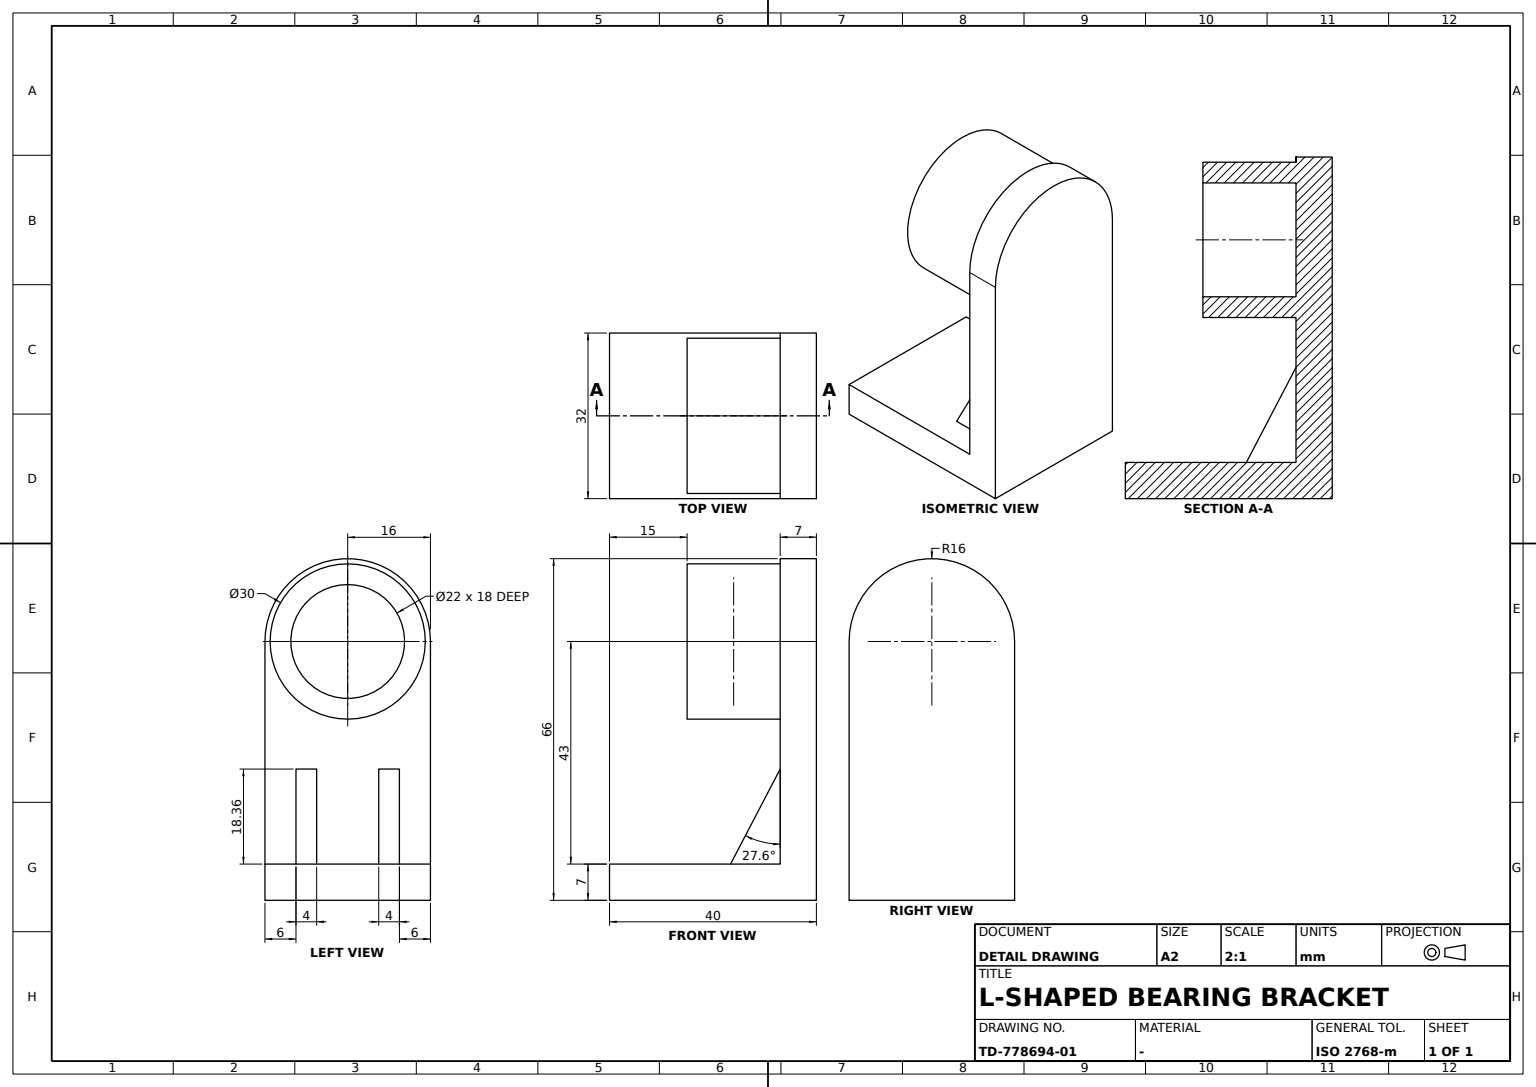
ISO-10303-21;
HEADER;
FILE_DESCRIPTION((''),'2;1');
FILE_NAME('','',(''),(''),'','','');
FILE_SCHEMA(('AUTOMOTIVE_DESIGN'));
ENDSEC;
DATA;
#1=APPLICATION_CONTEXT('');
#2=PRODUCT_CONTEXT('',#1,'mechanical');
#3=PRODUCT('','','',(#2));
#4=PRODUCT_DEFINITION_FORMATION('','',#3);
#5=PRODUCT_DEFINITION_CONTEXT('',#1,'design');
#6=PRODUCT_DEFINITION('','',#4,#5);
#7=PRODUCT_DEFINITION_SHAPE('','',#6);
#8=(LENGTH_UNIT()NAMED_UNIT(*)SI_UNIT(.MILLI.,.METRE.));
#9=(NAMED_UNIT(*)PLANE_ANGLE_UNIT()SI_UNIT($,.RADIAN.));
#10=(NAMED_UNIT(*)SI_UNIT($,.STERADIAN.)SOLID_ANGLE_UNIT());
#11=UNCERTAINTY_MEASURE_WITH_UNIT(LENGTH_MEASURE(0.005),#8,'distance_accuracy_value','');
#12=(GEOMETRIC_REPRESENTATION_CONTEXT(3)GLOBAL_UNCERTAINTY_ASSIGNED_CONTEXT((#11))GLOBAL_UNIT_ASSIGNED_CONTEXT((#8,#9,#10))REPRESENTATION_CONTEXT('',''));
#13=CARTESIAN_POINT('',(13.,0.,39.));
#14=VERTEX_POINT('',#13);
#15=CARTESIAN_POINT('',(13.,0.,50.));
#16=DIRECTION('',(1.,0.,0.));
#17=DIRECTION('',(0.,0.,-1.));
#18=AXIS2_PLACEMENT_3D('',#15,#16,#17);
#19=CIRCLE('',#18,11.);
#20=EDGE_CURVE('',#14,#14,#19,.F.);
#21=ORIENTED_EDGE('',*,*,#20,.T.);
#22=EDGE_LOOP('',(#21));
#23=FACE_BOUND('',#22,.T.);
#24=CARTESIAN_POINT('',(13.,0.,0.));
#25=DIRECTION('',(0.,1.,0.));
#26=AXIS2_PLACEMENT_3D('',#24,#16,#25);
#27=PLANE('',#26);
#28=ADVANCED_FACE('',(#23),#27,.F.);
#29=CARTESIAN_POINT('',(13.,-10.,7.));
#30=VERTEX_POINT('',#29);
#31=CARTESIAN_POINT('',(3.401389,-10.,7.));
#32=VERTEX_POINT('',#31);
#33=CARTESIAN_POINT('',(0.,-10.,7.));
#34=DIRECTION('',(-1.,0.,0.));
#35=VECTOR('',#34,1000.);
#36=LINE('',#33,#35);
#37=EDGE_CURVE('',#30,#32,#36,.T.);
#38=ORIENTED_EDGE('',*,*,#37,.F.);
#39=CARTESIAN_POINT('',(13.,-10.,25.357214));
#40=VERTEX_POINT('',#39);
#41=CARTESIAN_POINT('',(13.,-10.,0.));
#42=VECTOR('',#17,1000.);
#43=LINE('',#41,#42);
#44=EDGE_CURVE('',#40,#30,#43,.T.);
#45=ORIENTED_EDGE('',*,*,#44,.F.);
#46=DIRECTION('',(0.463360165,0.,0.88617005));
#47=VECTOR('',#46,1000.);
#48=LINE('',#31,#47);
#49=EDGE_CURVE('',#32,#40,#48,.T.);
#50=ORIENTED_EDGE('',*,*,#49,.F.);
#51=EDGE_LOOP('',(#38,#45,#50));
#52=FACE_BOUND('',#51,.T.);
#53=CARTESIAN_POINT('',(0.,-10.,0.));
#54=AXIS2_PLACEMENT_3D('',#53,#25,#34);
#55=PLANE('',#54);
#56=ADVANCED_FACE('',(#52),#55,.F.);
#57=CARTESIAN_POINT('',(20.,16.,0.));
#58=VERTEX_POINT('',#57);
#59=CARTESIAN_POINT('',(20.,-16.,0.));
#60=VERTEX_POINT('',#59);
#61=CARTESIAN_POINT('',(20.,0.,0.));
#62=DIRECTION('',(0.,-1.,0.));
#63=VECTOR('',#62,1000.);
#64=LINE('',#61,#63);
#65=EDGE_CURVE('',#58,#60,#64,.T.);
#66=ORIENTED_EDGE('',*,*,#65,.F.);
#67=CARTESIAN_POINT('',(20.,16.,50.));
#68=VERTEX_POINT('',#67);
#69=DIRECTION('',(0.,0.,1.));
#70=VECTOR('',#69,1000.);
#71=LINE('',#57,#70);
#72=EDGE_CURVE('',#58,#68,#71,.T.);
#73=ORIENTED_EDGE('',*,*,#72,.T.);
#74=CARTESIAN_POINT('',(20.,-16.,50.));
#75=VERTEX_POINT('',#74);
#76=CARTESIAN_POINT('',(20.,0.,50.));
#77=AXIS2_PLACEMENT_3D('',#76,#34,#69);
#78=CIRCLE('',#77,16.);
#79=EDGE_CURVE('',#68,#75,#78,.F.);
#80=ORIENTED_EDGE('',*,*,#79,.T.);
#81=LINE('',#59,#70);
#82=EDGE_CURVE('',#60,#75,#81,.T.);
#83=ORIENTED_EDGE('',*,*,#82,.F.);
#84=EDGE_LOOP('',(#66,#73,#80,#83));
#85=FACE_BOUND('',#84,.T.);
#86=AXIS2_PLACEMENT_3D('',#57,#34,#62);
#87=PLANE('',#86);
#88=ADVANCED_FACE('',(#85),#87,.F.);
#89=CARTESIAN_POINT('',(-20.,16.,0.));
#90=VERTEX_POINT('',#89);
#91=CARTESIAN_POINT('',(0.,16.,0.));
#92=VECTOR('',#16,1000.);
#93=LINE('',#91,#92);
#94=EDGE_CURVE('',#90,#58,#93,.T.);
#95=ORIENTED_EDGE('',*,*,#94,.F.);
#96=CARTESIAN_POINT('',(-20.,16.,7.));
#97=VERTEX_POINT('',#96);
#98=LINE('',#89,#70);
#99=EDGE_CURVE('',#90,#97,#98,.T.);
#100=ORIENTED_EDGE('',*,*,#99,.T.);
#101=CARTESIAN_POINT('',(13.,16.,7.));
#102=VERTEX_POINT('',#101);
#103=CARTESIAN_POINT('',(0.,16.,7.));
#104=LINE('',#103,#92);
#105=EDGE_CURVE('',#97,#102,#104,.T.);
#106=ORIENTED_EDGE('',*,*,#105,.T.);
#107=CARTESIAN_POINT('',(13.,16.,50.));
#108=VERTEX_POINT('',#107);
#109=CARTESIAN_POINT('',(13.,16.,0.));
#110=LINE('',#109,#70);
#111=EDGE_CURVE('',#102,#108,#110,.T.);
#112=ORIENTED_EDGE('',*,*,#111,.T.);
#113=CARTESIAN_POINT('',(16.5,16.,50.));
#114=LINE('',#113,#92);
#115=EDGE_CURVE('',#68,#108,#114,.F.);
#116=ORIENTED_EDGE('',*,*,#115,.F.);
#117=ORIENTED_EDGE('',*,*,#72,.F.);
#118=EDGE_LOOP('',(#95,#100,#106,#112,#116,#117));
#119=FACE_BOUND('',#118,.T.);
#120=AXIS2_PLACEMENT_3D('',#89,#62,#16);
#121=PLANE('',#120);
#122=ADVANCED_FACE('',(#119),#121,.F.);
#123=CARTESIAN_POINT('',(13.,0.,35.));
#124=VERTEX_POINT('',#123);
#125=CIRCLE('',#18,15.);
#126=EDGE_CURVE('',#124,#124,#125,.F.);
#127=ORIENTED_EDGE('',*,*,#126,.T.);
#128=EDGE_LOOP('',(#127));
#129=FACE_BOUND('',#128,.T.);
#130=CARTESIAN_POINT('',(-5.,0.,65.));
#131=VERTEX_POINT('',#130);
#132=CARTESIAN_POINT('',(-5.,0.,50.));
#133=AXIS2_PLACEMENT_3D('',#132,#34,#69);
#134=CIRCLE('',#133,15.);
#135=EDGE_CURVE('',#131,#131,#134,.T.);
#136=ORIENTED_EDGE('',*,*,#135,.F.);
#137=EDGE_LOOP('',(#136));
#138=FACE_BOUND('',#137,.T.);
#139=CARTESIAN_POINT('',(4.,0.,50.));
#140=AXIS2_PLACEMENT_3D('',#139,#34,#62);
#141=CYLINDRICAL_SURFACE('',#140,15.);
#142=ADVANCED_FACE('',(#129,#138),#141,.T.);
#143=CARTESIAN_POINT('',(13.,-6.,25.357214));
#144=VERTEX_POINT('',#143);
#145=CARTESIAN_POINT('',(13.,10.,25.357214));
#146=LINE('',#145,#63);
#147=EDGE_CURVE('',#144,#40,#146,.T.);
#148=ORIENTED_EDGE('',*,*,#147,.F.);
#149=CARTESIAN_POINT('',(3.401389,-6.,7.));
#150=VERTEX_POINT('',#149);
#151=LINE('',#149,#47);
#152=EDGE_CURVE('',#150,#144,#151,.T.);
#153=ORIENTED_EDGE('',*,*,#152,.F.);
#154=CARTESIAN_POINT('',(3.401389,10.,7.));
#155=LINE('',#154,#63);
#156=EDGE_CURVE('',#150,#32,#155,.T.);
#157=ORIENTED_EDGE('',*,*,#156,.T.);
#158=ORIENTED_EDGE('',*,*,#49,.T.);
#159=EDGE_LOOP('',(#148,#153,#157,#158));
#160=FACE_BOUND('',#159,.T.);
#161=DIRECTION('',(0.88617005,0.,-0.463360165));
#162=AXIS2_PLACEMENT_3D('',#154,#161,#46);
#163=PLANE('',#162);
#164=ADVANCED_FACE('',(#160),#163,.F.);
#165=CARTESIAN_POINT('',(13.,-6.,7.));
#166=VERTEX_POINT('',#165);
#167=CARTESIAN_POINT('',(0.,-6.,7.));
#168=LINE('',#167,#35);
#169=EDGE_CURVE('',#166,#150,#168,.T.);
#170=ORIENTED_EDGE('',*,*,#169,.F.);
#171=CARTESIAN_POINT('',(13.,6.,7.));
#172=VERTEX_POINT('',#171);
#173=CARTESIAN_POINT('',(13.,0.,7.));
#174=VECTOR('',#25,1000.);
#175=LINE('',#173,#174);
#176=EDGE_CURVE('',#166,#172,#175,.T.);
#177=ORIENTED_EDGE('',*,*,#176,.T.);
#178=CARTESIAN_POINT('',(3.401389,6.,7.));
#179=VERTEX_POINT('',#178);
#180=CARTESIAN_POINT('',(0.,6.,7.));
#181=LINE('',#180,#35);
#182=EDGE_CURVE('',#172,#179,#181,.T.);
#183=ORIENTED_EDGE('',*,*,#182,.T.);
#184=VERTEX_POINT('',#154);
#185=EDGE_CURVE('',#184,#179,#155,.T.);
#186=ORIENTED_EDGE('',*,*,#185,.F.);
#187=CARTESIAN_POINT('',(13.,10.,7.));
#188=VERTEX_POINT('',#187);
#189=CARTESIAN_POINT('',(0.,10.,7.));
#190=LINE('',#189,#35);
#191=EDGE_CURVE('',#188,#184,#190,.T.);
#192=ORIENTED_EDGE('',*,*,#191,.F.);
#193=EDGE_CURVE('',#188,#102,#175,.T.);
#194=ORIENTED_EDGE('',*,*,#193,.T.);
#195=ORIENTED_EDGE('',*,*,#105,.F.);
#196=CARTESIAN_POINT('',(-20.,-16.,7.));
#197=VERTEX_POINT('',#196);
#198=CARTESIAN_POINT('',(-20.,0.,7.));
#199=LINE('',#198,#174);
#200=EDGE_CURVE('',#197,#97,#199,.T.);
#201=ORIENTED_EDGE('',*,*,#200,.F.);
#202=CARTESIAN_POINT('',(13.,-16.,7.));
#203=VERTEX_POINT('',#202);
#204=CARTESIAN_POINT('',(0.,-16.,7.));
#205=LINE('',#204,#35);
#206=EDGE_CURVE('',#203,#197,#205,.T.);
#207=ORIENTED_EDGE('',*,*,#206,.F.);
#208=EDGE_CURVE('',#203,#30,#175,.T.);
#209=ORIENTED_EDGE('',*,*,#208,.T.);
#210=ORIENTED_EDGE('',*,*,#37,.T.);
#211=ORIENTED_EDGE('',*,*,#156,.F.);
#212=EDGE_LOOP('',(#170,#177,#183,#186,#192,#194,#195,#201,#207,#209,#210,#211));
#213=FACE_BOUND('',#212,.T.);
#214=CARTESIAN_POINT('',(0.,0.,7.));
#215=AXIS2_PLACEMENT_3D('',#214,#69,#16);
#216=PLANE('',#215);
#217=ADVANCED_FACE('',(#213),#216,.T.);
#218=ORIENTED_EDGE('',*,*,#94,.T.);
#219=ORIENTED_EDGE('',*,*,#65,.T.);
#220=CARTESIAN_POINT('',(-20.,-16.,0.));
#221=VERTEX_POINT('',#220);
#222=CARTESIAN_POINT('',(0.,-16.,0.));
#223=LINE('',#222,#35);
#224=EDGE_CURVE('',#60,#221,#223,.T.);
#225=ORIENTED_EDGE('',*,*,#224,.T.);
#226=CARTESIAN_POINT('',(-20.,0.,0.));
#227=LINE('',#226,#174);
#228=EDGE_CURVE('',#221,#90,#227,.T.);
#229=ORIENTED_EDGE('',*,*,#228,.T.);
#230=EDGE_LOOP('',(#218,#219,#225,#229));
#231=FACE_BOUND('',#230,.T.);
#232=CARTESIAN_POINT('',(0.,0.,0.));
#233=AXIS2_PLACEMENT_3D('',#232,#69,#16);
#234=PLANE('',#233);
#235=ADVANCED_FACE('',(#231),#234,.F.);
#236=ORIENTED_EDGE('',*,*,#126,.F.);
#237=EDGE_LOOP('',(#236));
#238=FACE_BOUND('',#237,.T.);
#239=ORIENTED_EDGE('',*,*,#111,.F.);
#240=ORIENTED_EDGE('',*,*,#193,.F.);
#241=VERTEX_POINT('',#145);
#242=CARTESIAN_POINT('',(13.,10.,0.));
#243=LINE('',#242,#42);
#244=EDGE_CURVE('',#241,#188,#243,.T.);
#245=ORIENTED_EDGE('',*,*,#244,.F.);
#246=CARTESIAN_POINT('',(13.,6.,25.357214));
#247=VERTEX_POINT('',#246);
#248=EDGE_CURVE('',#241,#247,#146,.T.);
#249=ORIENTED_EDGE('',*,*,#248,.T.);
#250=CARTESIAN_POINT('',(13.,6.,0.));
#251=LINE('',#250,#42);
#252=EDGE_CURVE('',#247,#172,#251,.T.);
#253=ORIENTED_EDGE('',*,*,#252,.T.);
#254=ORIENTED_EDGE('',*,*,#176,.F.);
#255=CARTESIAN_POINT('',(13.,-6.,0.));
#256=LINE('',#255,#42);
#257=EDGE_CURVE('',#144,#166,#256,.T.);
#258=ORIENTED_EDGE('',*,*,#257,.F.);
#259=ORIENTED_EDGE('',*,*,#147,.T.);
#260=ORIENTED_EDGE('',*,*,#44,.T.);
#261=ORIENTED_EDGE('',*,*,#208,.F.);
#262=CARTESIAN_POINT('',(13.,-16.,50.));
#263=VERTEX_POINT('',#262);
#264=CARTESIAN_POINT('',(13.,-16.,0.));
#265=LINE('',#264,#70);
#266=EDGE_CURVE('',#203,#263,#265,.T.);
#267=ORIENTED_EDGE('',*,*,#266,.T.);
#268=CIRCLE('',#18,16.);
#269=EDGE_CURVE('',#108,#263,#268,.T.);
#270=ORIENTED_EDGE('',*,*,#269,.F.);
#271=EDGE_LOOP('',(#239,#240,#245,#249,#253,#254,#258,#259,#260,#261,#267,#270));
#272=FACE_BOUND('',#271,.T.);
#273=ADVANCED_FACE('',(#238,#272),#27,.F.);
#274=CARTESIAN_POINT('',(-5.,0.,61.));
#275=VERTEX_POINT('',#274);
#276=CIRCLE('',#133,11.);
#277=EDGE_CURVE('',#275,#275,#276,.T.);
#278=ORIENTED_EDGE('',*,*,#277,.T.);
#279=EDGE_LOOP('',(#278));
#280=FACE_BOUND('',#279,.T.);
#281=ORIENTED_EDGE('',*,*,#20,.F.);
#282=EDGE_LOOP('',(#281));
#283=FACE_BOUND('',#282,.T.);
#284=CYLINDRICAL_SURFACE('',#140,11.);
#285=ADVANCED_FACE('',(#280,#283),#284,.F.);
#286=ORIENTED_EDGE('',*,*,#152,.T.);
#287=ORIENTED_EDGE('',*,*,#257,.T.);
#288=ORIENTED_EDGE('',*,*,#169,.T.);
#289=EDGE_LOOP('',(#286,#287,#288));
#290=FACE_BOUND('',#289,.T.);
#291=CARTESIAN_POINT('',(0.,-6.,0.));
#292=AXIS2_PLACEMENT_3D('',#291,#25,#34);
#293=PLANE('',#292);
#294=ADVANCED_FACE('',(#290),#293,.T.);
#295=ORIENTED_EDGE('',*,*,#135,.T.);
#296=EDGE_LOOP('',(#295));
#297=FACE_BOUND('',#296,.T.);
#298=ORIENTED_EDGE('',*,*,#277,.F.);
#299=EDGE_LOOP('',(#298));
#300=FACE_BOUND('',#299,.T.);
#301=CARTESIAN_POINT('',(-5.,0.,0.));
#302=AXIS2_PLACEMENT_3D('',#301,#34,#62);
#303=PLANE('',#302);
#304=ADVANCED_FACE('',(#297,#300),#303,.T.);
#305=ORIENTED_EDGE('',*,*,#79,.F.);
#306=ORIENTED_EDGE('',*,*,#115,.T.);
#307=ORIENTED_EDGE('',*,*,#269,.T.);
#308=CARTESIAN_POINT('',(16.5,-16.,50.));
#309=LINE('',#308,#92);
#310=EDGE_CURVE('',#75,#263,#309,.F.);
#311=ORIENTED_EDGE('',*,*,#310,.F.);
#312=EDGE_LOOP('',(#305,#306,#307,#311));
#313=FACE_BOUND('',#312,.T.);
#314=CARTESIAN_POINT('',(16.5,0.,50.));
#315=AXIS2_PLACEMENT_3D('',#314,#16,#25);
#316=CYLINDRICAL_SURFACE('',#315,16.);
#317=ADVANCED_FACE('',(#313),#316,.T.);
#318=LINE('',#178,#47);
#319=EDGE_CURVE('',#179,#247,#318,.T.);
#320=ORIENTED_EDGE('',*,*,#319,.F.);
#321=ORIENTED_EDGE('',*,*,#182,.F.);
#322=ORIENTED_EDGE('',*,*,#252,.F.);
#323=EDGE_LOOP('',(#320,#321,#322));
#324=FACE_BOUND('',#323,.T.);
#325=CARTESIAN_POINT('',(0.,6.,0.));
#326=AXIS2_PLACEMENT_3D('',#325,#25,#34);
#327=PLANE('',#326);
#328=ADVANCED_FACE('',(#324),#327,.F.);
#329=LINE('',#154,#47);
#330=EDGE_CURVE('',#184,#241,#329,.T.);
#331=ORIENTED_EDGE('',*,*,#330,.F.);
#332=ORIENTED_EDGE('',*,*,#185,.T.);
#333=ORIENTED_EDGE('',*,*,#319,.T.);
#334=ORIENTED_EDGE('',*,*,#248,.F.);
#335=EDGE_LOOP('',(#331,#332,#333,#334));
#336=FACE_BOUND('',#335,.T.);
#337=ADVANCED_FACE('',(#336),#163,.F.);
#338=ORIENTED_EDGE('',*,*,#310,.T.);
#339=ORIENTED_EDGE('',*,*,#266,.F.);
#340=ORIENTED_EDGE('',*,*,#206,.T.);
#341=LINE('',#220,#70);
#342=EDGE_CURVE('',#221,#197,#341,.T.);
#343=ORIENTED_EDGE('',*,*,#342,.F.);
#344=ORIENTED_EDGE('',*,*,#224,.F.);
#345=ORIENTED_EDGE('',*,*,#82,.T.);
#346=EDGE_LOOP('',(#338,#339,#340,#343,#344,#345));
#347=FACE_BOUND('',#346,.T.);
#348=AXIS2_PLACEMENT_3D('',#59,#25,#34);
#349=PLANE('',#348);
#350=ADVANCED_FACE('',(#347),#349,.F.);
#351=ORIENTED_EDGE('',*,*,#99,.F.);
#352=ORIENTED_EDGE('',*,*,#228,.F.);
#353=ORIENTED_EDGE('',*,*,#342,.T.);
#354=ORIENTED_EDGE('',*,*,#200,.T.);
#355=EDGE_LOOP('',(#351,#352,#353,#354));
#356=FACE_BOUND('',#355,.T.);
#357=AXIS2_PLACEMENT_3D('',#220,#16,#25);
#358=PLANE('',#357);
#359=ADVANCED_FACE('',(#356),#358,.F.);
#360=ORIENTED_EDGE('',*,*,#191,.T.);
#361=ORIENTED_EDGE('',*,*,#330,.T.);
#362=ORIENTED_EDGE('',*,*,#244,.T.);
#363=EDGE_LOOP('',(#360,#361,#362));
#364=FACE_BOUND('',#363,.T.);
#365=CARTESIAN_POINT('',(0.,10.,0.));
#366=AXIS2_PLACEMENT_3D('',#365,#25,#34);
#367=PLANE('',#366);
#368=ADVANCED_FACE('',(#364),#367,.T.);
#369=CLOSED_SHELL('',(#28,#56,#88,#122,#142,#164,#217,#235,#273,#285,#294,#304,#317,#328,#337,#350,#359,#368));
#370=MANIFOLD_SOLID_BREP('',#369);
#371=ADVANCED_BREP_SHAPE_REPRESENTATION('',(#370),#12);
#372=SHAPE_DEFINITION_REPRESENTATION(#7,#371);
ENDSEC;
END-ISO-10303-21;
